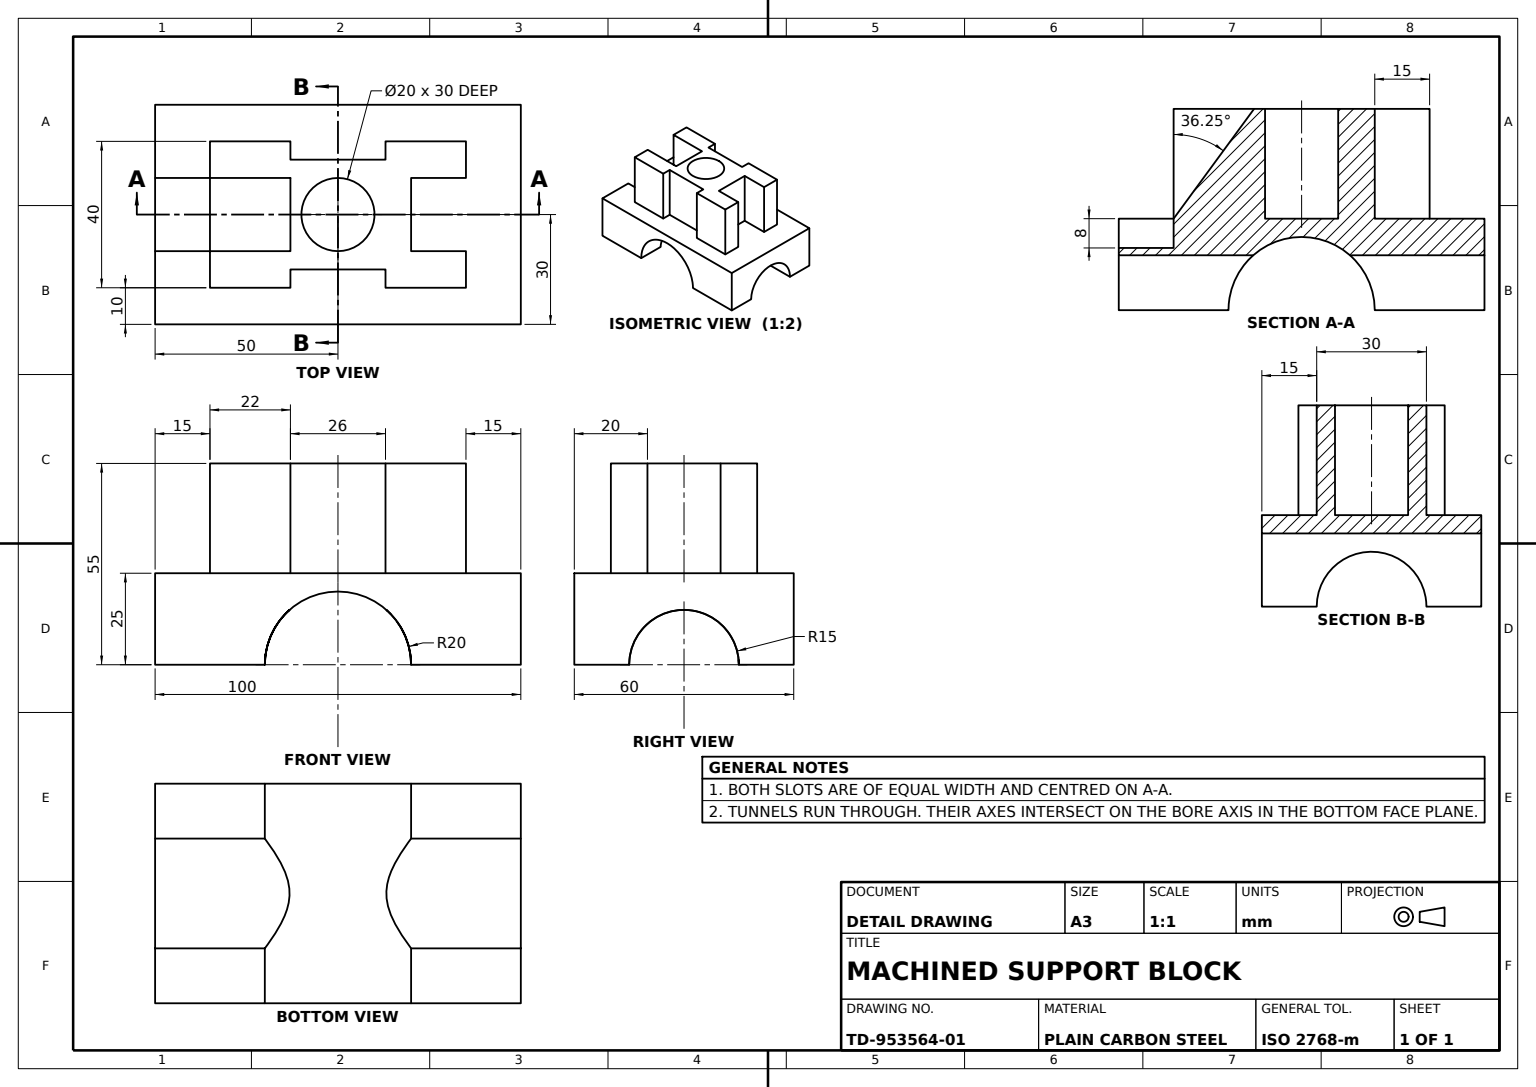
ISO-10303-21;
HEADER;
FILE_DESCRIPTION((''),'2;1');
FILE_NAME('','',(''),(''),'','','');
FILE_SCHEMA(('AUTOMOTIVE_DESIGN'));
ENDSEC;
DATA;
#1=APPLICATION_CONTEXT('');
#2=PRODUCT_CONTEXT('',#1,'mechanical');
#3=PRODUCT('','','',(#2));
#4=PRODUCT_DEFINITION_FORMATION('','',#3);
#5=PRODUCT_DEFINITION_CONTEXT('',#1,'design');
#6=PRODUCT_DEFINITION('','',#4,#5);
#7=PRODUCT_DEFINITION_SHAPE('','',#6);
#8=(LENGTH_UNIT()NAMED_UNIT(*)SI_UNIT(.MILLI.,.METRE.));
#9=(NAMED_UNIT(*)PLANE_ANGLE_UNIT()SI_UNIT($,.RADIAN.));
#10=(NAMED_UNIT(*)SI_UNIT($,.STERADIAN.)SOLID_ANGLE_UNIT());
#11=UNCERTAINTY_MEASURE_WITH_UNIT(LENGTH_MEASURE(1.E-05),#8,'distance_accuracy_value','');
#12=(GEOMETRIC_REPRESENTATION_CONTEXT(3)GLOBAL_UNCERTAINTY_ASSIGNED_CONTEXT((#11))GLOBAL_UNIT_ASSIGNED_CONTEXT((#8,#9,#10))REPRESENTATION_CONTEXT('',''));
#13=CARTESIAN_POINT('',(35.,42.5,20.));
#14=VERTEX_POINT('',#13);
#15=CARTESIAN_POINT('',(35.,12.5,20.));
#16=VERTEX_POINT('',#15);
#17=DIRECTION('',(0.,-1.,0.));
#18=VECTOR('',#17,1000.);
#19=LINE('',#13,#18);
#20=EDGE_CURVE('',#14,#16,#19,.T.);
#21=ORIENTED_EDGE('',*,*,#20,.F.);
#22=CARTESIAN_POINT('',(13.,42.5,20.));
#23=VERTEX_POINT('',#22);
#24=DIRECTION('',(1.,0.,0.));
#25=VECTOR('',#24,1000.);
#26=LINE('',#13,#25);
#27=EDGE_CURVE('',#23,#14,#26,.T.);
#28=ORIENTED_EDGE('',*,*,#27,.F.);
#29=CARTESIAN_POINT('',(13.,12.5,20.));
#30=VERTEX_POINT('',#29);
#31=LINE('',#22,#18);
#32=EDGE_CURVE('',#23,#30,#31,.T.);
#33=ORIENTED_EDGE('',*,*,#32,.T.);
#34=LINE('',#15,#25);
#35=EDGE_CURVE('',#30,#16,#34,.T.);
#36=ORIENTED_EDGE('',*,*,#35,.T.);
#37=EDGE_LOOP('',(#21,#28,#33,#36));
#38=FACE_OUTER_BOUND('',#37,.T.);
#39=DIRECTION('',(0.,0.,-1.));
#40=DIRECTION('',(-1.,0.,0.));
#41=AXIS2_PLACEMENT_3D('',#13,#39,#40);
#42=PLANE('',#41);
#43=ADVANCED_FACE('',(#38),#42,.F.);
#44=CARTESIAN_POINT('',(-35.,12.5,20.));
#45=VERTEX_POINT('',#44);
#46=CARTESIAN_POINT('',(-13.,12.5,20.));
#47=VERTEX_POINT('',#46);
#48=LINE('',#46,#25);
#49=EDGE_CURVE('',#45,#47,#48,.T.);
#50=ORIENTED_EDGE('',*,*,#49,.T.);
#51=CARTESIAN_POINT('',(-13.,42.5,20.));
#52=VERTEX_POINT('',#51);
#53=LINE('',#51,#18);
#54=EDGE_CURVE('',#52,#47,#53,.T.);
#55=ORIENTED_EDGE('',*,*,#54,.F.);
#56=CARTESIAN_POINT('',(-35.,42.5,20.));
#57=VERTEX_POINT('',#56);
#58=VECTOR('',#40,1000.);
#59=LINE('',#56,#58);
#60=EDGE_CURVE('',#52,#57,#59,.T.);
#61=ORIENTED_EDGE('',*,*,#60,.T.);
#62=LINE('',#44,#18);
#63=EDGE_CURVE('',#57,#45,#62,.T.);
#64=ORIENTED_EDGE('',*,*,#63,.T.);
#65=EDGE_LOOP('',(#50,#55,#61,#64));
#66=FACE_OUTER_BOUND('',#65,.T.);
#67=AXIS2_PLACEMENT_3D('',#51,#39,#40);
#68=PLANE('',#67);
#69=ADVANCED_FACE('',(#66),#68,.F.);
#70=CARTESIAN_POINT('',(35.,42.5,-10.));
#71=VERTEX_POINT('',#70);
#72=CARTESIAN_POINT('',(35.,12.5,-10.));
#73=VERTEX_POINT('',#72);
#74=LINE('',#70,#18);
#75=EDGE_CURVE('',#71,#73,#74,.T.);
#76=ORIENTED_EDGE('',*,*,#75,.F.);
#77=CARTESIAN_POINT('',(20.,42.5,-10.));
#78=VERTEX_POINT('',#77);
#79=LINE('',#77,#25);
#80=EDGE_CURVE('',#78,#71,#79,.T.);
#81=ORIENTED_EDGE('',*,*,#80,.F.);
#82=CARTESIAN_POINT('',(20.,12.5,-10.));
#83=VERTEX_POINT('',#82);
#84=LINE('',#77,#18);
#85=EDGE_CURVE('',#78,#83,#84,.T.);
#86=ORIENTED_EDGE('',*,*,#85,.T.);
#87=LINE('',#82,#25);
#88=EDGE_CURVE('',#83,#73,#87,.T.);
#89=ORIENTED_EDGE('',*,*,#88,.T.);
#90=EDGE_LOOP('',(#76,#81,#86,#89));
#91=FACE_OUTER_BOUND('',#90,.T.);
#92=AXIS2_PLACEMENT_3D('',#77,#39,#40);
#93=PLANE('',#92);
#94=ADVANCED_FACE('',(#91),#93,.F.);
#95=CARTESIAN_POINT('',(-20.,-12.5,30.));
#96=VERTEX_POINT('',#95);
#97=CARTESIAN_POINT('',(20.,-12.5,30.));
#98=VERTEX_POINT('',#97);
#99=CARTESIAN_POINT('',(0.,-12.5,30.));
#100=AXIS2_PLACEMENT_3D('',#99,#39,#24);
#101=CIRCLE('',#100,20.);
#102=EDGE_CURVE('',#96,#98,#101,.T.);
#103=ORIENTED_EDGE('',*,*,#102,.F.);
#104=CARTESIAN_POINT('',(-20.,-12.5,15.));
#105=VERTEX_POINT('',#104);
#106=VECTOR('',#39,1000.);
#107=LINE('',#95,#106);
#108=EDGE_CURVE('',#96,#105,#107,.T.);
#109=ORIENTED_EDGE('',*,*,#108,.T.);
#110=CARTESIAN_POINT('',(-20.,-12.5,-15.));
#111=VERTEX_POINT('',#110);
#112=CARTESIAN_POINT('',(-20.,-11.460012,15.));
#113=CARTESIAN_POINT('',(-19.91945,-10.444489,14.89307));
#114=CARTESIAN_POINT('',(-19.68971,-8.954901,14.583876));
#115=CARTESIAN_POINT('',(-19.594347,-8.461833,14.455074));
#116=CARTESIAN_POINT('',(-19.370481,-7.49703,14.150132));
#117=CARTESIAN_POINT('',(-19.243229,-7.02976,13.975697));
#118=CARTESIAN_POINT('',(-18.961995,-6.122842,13.585856));
#119=CARTESIAN_POINT('',(-18.807998,-5.683203,13.37044));
#120=CARTESIAN_POINT('',(-18.476456,-4.829922,12.899895));
#121=CARTESIAN_POINT('',(-18.297983,-4.414425,12.64341));
#122=CARTESIAN_POINT('',(-17.739419,-3.221867,11.825632));
#123=CARTESIAN_POINT('',(-17.337061,-2.498089,11.218166));
#124=CARTESIAN_POINT('',(-16.711435,-1.505414,10.214717));
#125=CARTESIAN_POINT('',(-16.498395,-1.18907,9.863302));
#126=CARTESIAN_POINT('',(-16.073156,-0.592531,9.134223));
#127=CARTESIAN_POINT('',(-15.861739,-0.31326,8.758001));
#128=CARTESIAN_POINT('',(-15.238528,0.470461,7.592364));
#129=CARTESIAN_POINT('',(-14.836864,0.921647,6.766908));
#130=CARTESIAN_POINT('',(-14.29593,1.489091,5.434909));
#131=CARTESIAN_POINT('',(-14.125386,1.660451,4.972426));
#132=CARTESIAN_POINT('',(-13.822168,1.956576,4.031229));
#133=CARTESIAN_POINT('',(-13.688686,2.082271,3.550951));
#134=CARTESIAN_POINT('',(-13.467259,2.28701,2.568307));
#135=CARTESIAN_POINT('',(-13.379218,2.366168,2.065023));
#136=CARTESIAN_POINT('',(-13.259474,2.473069,1.036579));
#137=CARTESIAN_POINT('',(-13.22921,2.4996,0.523513));
#138=CARTESIAN_POINT('',(-13.228313,2.500391,-0.500332));
#139=CARTESIAN_POINT('',(-13.257676,2.474649,-1.011111));
#140=CARTESIAN_POINT('',(-13.374088,2.370772,-2.030418));
#141=CARTESIAN_POINT('',(-13.461925,2.291862,-2.540716));
#142=CARTESIAN_POINT('',(-13.682828,2.087763,-3.528684));
#143=CARTESIAN_POINT('',(-13.816081,1.962383,-4.010379));
#144=CARTESIAN_POINT('',(-14.118367,1.667438,-4.952509));
#145=CARTESIAN_POINT('',(-14.288407,1.496778,-5.415214));
#146=CARTESIAN_POINT('',(-14.829898,0.929354,-6.752021));
#147=CARTESIAN_POINT('',(-15.232138,0.477984,-7.579673));
#148=CARTESIAN_POINT('',(-15.856074,-0.305885,-8.747768));
#149=CARTESIAN_POINT('',(-16.067715,-0.585187,-9.124663));
#150=CARTESIAN_POINT('',(-16.493336,-1.181692,-9.854854));
#151=CARTESIAN_POINT('',(-16.706461,-1.497879,-10.206576));
#152=CARTESIAN_POINT('',(-17.331547,-2.488635,-11.209639));
#153=CARTESIAN_POINT('',(-17.73267,-3.209534,-11.815456));
#154=CARTESIAN_POINT('',(-18.288634,-4.393461,-12.629864));
#155=CARTESIAN_POINT('',(-18.466869,-4.806673,-12.886183));
#156=CARTESIAN_POINT('',(-18.801726,-5.665702,-13.361638));
#157=CARTESIAN_POINT('',(-18.956617,-6.106875,-13.578352));
#158=CARTESIAN_POINT('',(-19.238591,-7.013474,-13.969314));
#159=CARTESIAN_POINT('',(-19.365686,-7.478895,-14.143566));
#160=CARTESIAN_POINT('',(-19.588837,-8.435671,-14.447602));
#161=CARTESIAN_POINT('',(-19.685272,-8.929505,-14.57789));
#162=CARTESIAN_POINT('',(-19.91921,-10.436366,-14.892772));
#163=CARTESIAN_POINT('',(-20.,-11.458775,-15.));
#164=B_SPLINE_CURVE_WITH_KNOTS('',3,(#104,#112,#113,#114,#115,#116,#117,#118,#119,#120,#121,#122,#123,#124,#125,#126,#127,#128,#129,#130,#131,#132,#133,#134,#135,#136,#137,#138,#139,#140,#141,#142,#143,#144,#145,#146,#147,#148,#149,#150,#151,#152,#153,#154,#155,#156,#157,#158,#159,#160,#161,#162,#163,#110),.UNSPECIFIED.,.F.,.F.,(4,2,2,2,2,2,2,2,2,2,2,2,2,2,2,2,2,2,2,2,2,2,2,2,2,2,4),(0.,0.003069136,0.004603704,0.006138272,0.00767284,0.009207408,0.012276544,0.013811112,0.01534568,0.018414816,0.019949384,0.021483952,0.02301852,0.024553088,0.026087656,0.027622224,0.029156792,0.03069136,0.033760496,0.035295064,0.036829632,0.039898768,0.041433336,0.042967904,0.044502472,0.04603704,0.049106176),.UNSPECIFIED.);
#165=EDGE_CURVE('',#105,#111,#164,.T.);
#166=ORIENTED_EDGE('',*,*,#165,.T.);
#167=CARTESIAN_POINT('',(-20.,-12.5,-30.));
#168=VERTEX_POINT('',#167);
#169=EDGE_CURVE('',#111,#168,#107,.T.);
#170=ORIENTED_EDGE('',*,*,#169,.T.);
#171=CARTESIAN_POINT('',(20.,-12.5,-30.));
#172=VERTEX_POINT('',#171);
#173=CARTESIAN_POINT('',(0.,-12.5,-30.));
#174=AXIS2_PLACEMENT_3D('',#173,#39,#24);
#175=CIRCLE('',#174,20.);
#176=EDGE_CURVE('',#168,#172,#175,.T.);
#177=ORIENTED_EDGE('',*,*,#176,.T.);
#178=CARTESIAN_POINT('',(20.,-12.5,-15.));
#179=VERTEX_POINT('',#178);
#180=LINE('',#97,#106);
#181=EDGE_CURVE('',#179,#172,#180,.T.);
#182=ORIENTED_EDGE('',*,*,#181,.F.);
#183=CARTESIAN_POINT('',(20.,-12.5,15.));
#184=VERTEX_POINT('',#183);
#185=CARTESIAN_POINT('',(20.,-11.460012,-15.));
#186=CARTESIAN_POINT('',(19.91945,-10.444489,-14.89307));
#187=CARTESIAN_POINT('',(19.68971,-8.954901,-14.583876));
#188=CARTESIAN_POINT('',(19.594347,-8.461833,-14.455074));
#189=CARTESIAN_POINT('',(19.370481,-7.49703,-14.150132));
#190=CARTESIAN_POINT('',(19.243229,-7.02976,-13.975697));
#191=CARTESIAN_POINT('',(18.961995,-6.122842,-13.585856));
#192=CARTESIAN_POINT('',(18.807998,-5.683203,-13.37044));
#193=CARTESIAN_POINT('',(18.476456,-4.829922,-12.899895));
#194=CARTESIAN_POINT('',(18.297983,-4.414425,-12.64341));
#195=CARTESIAN_POINT('',(17.739419,-3.221867,-11.825632));
#196=CARTESIAN_POINT('',(17.337061,-2.498089,-11.218166));
#197=CARTESIAN_POINT('',(16.711435,-1.505414,-10.214717));
#198=CARTESIAN_POINT('',(16.498395,-1.18907,-9.863302));
#199=CARTESIAN_POINT('',(16.073156,-0.592531,-9.134223));
#200=CARTESIAN_POINT('',(15.861739,-0.31326,-8.758001));
#201=CARTESIAN_POINT('',(15.238528,0.470461,-7.592364));
#202=CARTESIAN_POINT('',(14.836864,0.921647,-6.766908));
#203=CARTESIAN_POINT('',(14.29593,1.489091,-5.434909));
#204=CARTESIAN_POINT('',(14.125386,1.660451,-4.972426));
#205=CARTESIAN_POINT('',(13.822168,1.956576,-4.031229));
#206=CARTESIAN_POINT('',(13.688686,2.082271,-3.550951));
#207=CARTESIAN_POINT('',(13.467259,2.28701,-2.568307));
#208=CARTESIAN_POINT('',(13.379218,2.366168,-2.065023));
#209=CARTESIAN_POINT('',(13.259474,2.473069,-1.036579));
#210=CARTESIAN_POINT('',(13.22921,2.4996,-0.523513));
#211=CARTESIAN_POINT('',(13.228313,2.500391,0.500332));
#212=CARTESIAN_POINT('',(13.257676,2.474649,1.011111));
#213=CARTESIAN_POINT('',(13.374088,2.370772,2.030418));
#214=CARTESIAN_POINT('',(13.461925,2.291862,2.540716));
#215=CARTESIAN_POINT('',(13.682828,2.087763,3.528684));
#216=CARTESIAN_POINT('',(13.816081,1.962383,4.010379));
#217=CARTESIAN_POINT('',(14.118367,1.667438,4.952509));
#218=CARTESIAN_POINT('',(14.288407,1.496778,5.415214));
#219=CARTESIAN_POINT('',(14.829898,0.929354,6.752021));
#220=CARTESIAN_POINT('',(15.232138,0.477984,7.579673));
#221=CARTESIAN_POINT('',(15.856074,-0.305885,8.747768));
#222=CARTESIAN_POINT('',(16.067715,-0.585187,9.124663));
#223=CARTESIAN_POINT('',(16.493336,-1.181692,9.854854));
#224=CARTESIAN_POINT('',(16.706461,-1.497879,10.206576));
#225=CARTESIAN_POINT('',(17.331547,-2.488635,11.209639));
#226=CARTESIAN_POINT('',(17.73267,-3.209534,11.815456));
#227=CARTESIAN_POINT('',(18.288634,-4.393461,12.629864));
#228=CARTESIAN_POINT('',(18.466869,-4.806673,12.886183));
#229=CARTESIAN_POINT('',(18.801726,-5.665702,13.361638));
#230=CARTESIAN_POINT('',(18.956617,-6.106875,13.578352));
#231=CARTESIAN_POINT('',(19.238591,-7.013474,13.969314));
#232=CARTESIAN_POINT('',(19.365686,-7.478895,14.143566));
#233=CARTESIAN_POINT('',(19.588837,-8.435671,14.447602));
#234=CARTESIAN_POINT('',(19.685272,-8.929505,14.57789));
#235=CARTESIAN_POINT('',(19.91921,-10.436366,14.892772));
#236=CARTESIAN_POINT('',(20.,-11.458775,15.));
#237=B_SPLINE_CURVE_WITH_KNOTS('',3,(#178,#185,#186,#187,#188,#189,#190,#191,#192,#193,#194,#195,#196,#197,#198,#199,#200,#201,#202,#203,#204,#205,#206,#207,#208,#209,#210,#211,#212,#213,#214,#215,#216,#217,#218,#219,#220,#221,#222,#223,#224,#225,#226,#227,#228,#229,#230,#231,#232,#233,#234,#235,#236,#183),.UNSPECIFIED.,.F.,.F.,(4,2,2,2,2,2,2,2,2,2,2,2,2,2,2,2,2,2,2,2,2,2,2,2,2,2,4),(0.,0.003069136,0.004603704,0.006138272,0.00767284,0.009207408,0.012276544,0.013811112,0.01534568,0.018414816,0.019949384,0.021483952,0.02301852,0.024553088,0.026087656,0.027622224,0.029156792,0.03069136,0.033760496,0.035295064,0.036829632,0.039898768,0.041433336,0.042967904,0.044502472,0.04603704,0.049106176),.UNSPECIFIED.);
#238=EDGE_CURVE('',#179,#184,#237,.T.);
#239=ORIENTED_EDGE('',*,*,#238,.T.);
#240=EDGE_CURVE('',#98,#184,#180,.T.);
#241=ORIENTED_EDGE('',*,*,#240,.F.);
#242=EDGE_LOOP('',(#103,#109,#166,#170,#177,#182,#239,#241));
#243=FACE_OUTER_BOUND('',#242,.T.);
#244=AXIS2_PLACEMENT_3D('',#99,#39,#40);
#245=CYLINDRICAL_SURFACE('',#244,20.);
#246=ADVANCED_FACE('',(#243),#245,.F.);
#247=CARTESIAN_POINT('',(-13.,42.5,-20.));
#248=VERTEX_POINT('',#247);
#249=CARTESIAN_POINT('',(-13.,12.5,-20.));
#250=VERTEX_POINT('',#249);
#251=LINE('',#247,#18);
#252=EDGE_CURVE('',#248,#250,#251,.T.);
#253=ORIENTED_EDGE('',*,*,#252,.T.);
#254=CARTESIAN_POINT('',(-35.,12.5,-20.));
#255=VERTEX_POINT('',#254);
#256=LINE('',#249,#58);
#257=EDGE_CURVE('',#250,#255,#256,.T.);
#258=ORIENTED_EDGE('',*,*,#257,.T.);
#259=CARTESIAN_POINT('',(-35.,42.5,-20.));
#260=VERTEX_POINT('',#259);
#261=LINE('',#259,#18);
#262=EDGE_CURVE('',#260,#255,#261,.T.);
#263=ORIENTED_EDGE('',*,*,#262,.F.);
#264=LINE('',#247,#58);
#265=EDGE_CURVE('',#248,#260,#264,.T.);
#266=ORIENTED_EDGE('',*,*,#265,.F.);
#267=EDGE_LOOP('',(#253,#258,#263,#266));
#268=FACE_OUTER_BOUND('',#267,.T.);
#269=DIRECTION('',(0.,0.,1.));
#270=AXIS2_PLACEMENT_3D('',#247,#269,#24);
#271=PLANE('',#270);
#272=ADVANCED_FACE('',(#268),#271,.F.);
#273=CARTESIAN_POINT('',(-13.,42.5,15.));
#274=VERTEX_POINT('',#273);
#275=CARTESIAN_POINT('',(13.,42.5,15.));
#276=VERTEX_POINT('',#275);
#277=LINE('',#275,#25);
#278=EDGE_CURVE('',#274,#276,#277,.T.);
#279=ORIENTED_EDGE('',*,*,#278,.F.);
#280=CARTESIAN_POINT('',(-13.,12.5,15.));
#281=VERTEX_POINT('',#280);
#282=LINE('',#273,#18);
#283=EDGE_CURVE('',#274,#281,#282,.T.);
#284=ORIENTED_EDGE('',*,*,#283,.T.);
#285=CARTESIAN_POINT('',(13.,12.5,15.));
#286=VERTEX_POINT('',#285);
#287=LINE('',#285,#25);
#288=EDGE_CURVE('',#281,#286,#287,.T.);
#289=ORIENTED_EDGE('',*,*,#288,.T.);
#290=LINE('',#275,#18);
#291=EDGE_CURVE('',#276,#286,#290,.T.);
#292=ORIENTED_EDGE('',*,*,#291,.F.);
#293=EDGE_LOOP('',(#279,#284,#289,#292));
#294=FACE_OUTER_BOUND('',#293,.T.);
#295=AXIS2_PLACEMENT_3D('',#275,#39,#40);
#296=PLANE('',#295);
#297=ADVANCED_FACE('',(#294),#296,.F.);
#298=CARTESIAN_POINT('',(50.,-12.5,30.));
#299=VERTEX_POINT('',#298);
#300=CARTESIAN_POINT('',(50.,12.5,30.));
#301=VERTEX_POINT('',#300);
#302=DIRECTION('',(0.,1.,0.));
#303=VECTOR('',#302,1000.);
#304=LINE('',#300,#303);
#305=EDGE_CURVE('',#299,#301,#304,.T.);
#306=ORIENTED_EDGE('',*,*,#305,.T.);
#307=CARTESIAN_POINT('',(-50.,12.5,30.));
#308=VERTEX_POINT('',#307);
#309=LINE('',#307,#58);
#310=EDGE_CURVE('',#301,#308,#309,.T.);
#311=ORIENTED_EDGE('',*,*,#310,.T.);
#312=CARTESIAN_POINT('',(-50.,-12.5,30.));
#313=VERTEX_POINT('',#312);
#314=LINE('',#307,#18);
#315=EDGE_CURVE('',#308,#313,#314,.T.);
#316=ORIENTED_EDGE('',*,*,#315,.T.);
#317=LINE('',#312,#25);
#318=EDGE_CURVE('',#313,#96,#317,.T.);
#319=ORIENTED_EDGE('',*,*,#318,.T.);
#320=ORIENTED_EDGE('',*,*,#102,.T.);
#321=LINE('',#97,#25);
#322=EDGE_CURVE('',#98,#299,#321,.T.);
#323=ORIENTED_EDGE('',*,*,#322,.T.);
#324=EDGE_LOOP('',(#306,#311,#316,#319,#320,#323));
#325=FACE_OUTER_BOUND('',#324,.T.);
#326=AXIS2_PLACEMENT_3D('',#99,#269,#24);
#327=PLANE('',#326);
#328=ADVANCED_FACE('',(#325),#327,.T.);
#329=CARTESIAN_POINT('',(35.,12.5,-20.));
#330=VERTEX_POINT('',#329);
#331=LINE('',#72,#106);
#332=EDGE_CURVE('',#73,#330,#331,.T.);
#333=ORIENTED_EDGE('',*,*,#332,.T.);
#334=CARTESIAN_POINT('',(35.,42.5,-20.));
#335=VERTEX_POINT('',#334);
#336=LINE('',#334,#18);
#337=EDGE_CURVE('',#335,#330,#336,.T.);
#338=ORIENTED_EDGE('',*,*,#337,.F.);
#339=LINE('',#70,#106);
#340=EDGE_CURVE('',#71,#335,#339,.T.);
#341=ORIENTED_EDGE('',*,*,#340,.F.);
#342=ORIENTED_EDGE('',*,*,#75,.T.);
#343=EDGE_LOOP('',(#333,#338,#341,#342));
#344=FACE_OUTER_BOUND('',#343,.T.);
#345=AXIS2_PLACEMENT_3D('',#70,#40,#269);
#346=PLANE('',#345);
#347=ADVANCED_FACE('',(#344),#346,.F.);
#348=ORIENTED_EDGE('',*,*,#165,.F.);
#349=CARTESIAN_POINT('',(-50.,-12.5,15.));
#350=VERTEX_POINT('',#349);
#351=CARTESIAN_POINT('',(50.,-12.5,15.));
#352=LINE('',#351,#58);
#353=EDGE_CURVE('',#105,#350,#352,.T.);
#354=ORIENTED_EDGE('',*,*,#353,.T.);
#355=CARTESIAN_POINT('',(-50.,-12.5,-15.));
#356=VERTEX_POINT('',#355);
#357=CARTESIAN_POINT('',(-50.,-12.5,0.));
#358=AXIS2_PLACEMENT_3D('',#357,#40,#269);
#359=CIRCLE('',#358,15.);
#360=EDGE_CURVE('',#350,#356,#359,.T.);
#361=ORIENTED_EDGE('',*,*,#360,.T.);
#362=CARTESIAN_POINT('',(50.,-12.5,-15.));
#363=LINE('',#362,#58);
#364=EDGE_CURVE('',#111,#356,#363,.T.);
#365=ORIENTED_EDGE('',*,*,#364,.F.);
#366=EDGE_LOOP('',(#348,#354,#361,#365));
#367=FACE_OUTER_BOUND('',#366,.T.);
#368=CARTESIAN_POINT('',(50.,-12.5,0.));
#369=AXIS2_PLACEMENT_3D('',#368,#40,#269);
#370=CYLINDRICAL_SURFACE('',#369,15.);
#371=ADVANCED_FACE('',(#367),#370,.F.);
#372=ORIENTED_EDGE('',*,*,#20,.T.);
#373=CARTESIAN_POINT('',(35.,12.5,10.));
#374=VERTEX_POINT('',#373);
#375=LINE('',#373,#106);
#376=EDGE_CURVE('',#16,#374,#375,.T.);
#377=ORIENTED_EDGE('',*,*,#376,.T.);
#378=CARTESIAN_POINT('',(35.,42.5,10.));
#379=VERTEX_POINT('',#378);
#380=LINE('',#378,#18);
#381=EDGE_CURVE('',#379,#374,#380,.T.);
#382=ORIENTED_EDGE('',*,*,#381,.F.);
#383=LINE('',#378,#106);
#384=EDGE_CURVE('',#14,#379,#383,.T.);
#385=ORIENTED_EDGE('',*,*,#384,.F.);
#386=EDGE_LOOP('',(#372,#377,#382,#385));
#387=FACE_OUTER_BOUND('',#386,.T.);
#388=AXIS2_PLACEMENT_3D('',#378,#40,#269);
#389=PLANE('',#388);
#390=ADVANCED_FACE('',(#387),#389,.F.);
#391=CARTESIAN_POINT('',(-35.,12.5,-10.));
#392=VERTEX_POINT('',#391);
#393=CARTESIAN_POINT('',(-35.,4.5,-10.));
#394=VERTEX_POINT('',#393);
#395=LINE('',#393,#18);
#396=EDGE_CURVE('',#392,#394,#395,.T.);
#397=ORIENTED_EDGE('',*,*,#396,.F.);
#398=CARTESIAN_POINT('',(-50.,12.5,-10.));
#399=VERTEX_POINT('',#398);
#400=LINE('',#391,#58);
#401=EDGE_CURVE('',#392,#399,#400,.T.);
#402=ORIENTED_EDGE('',*,*,#401,.T.);
#403=CARTESIAN_POINT('',(-50.,4.5,-10.));
#404=VERTEX_POINT('',#403);
#405=LINE('',#403,#18);
#406=EDGE_CURVE('',#399,#404,#405,.T.);
#407=ORIENTED_EDGE('',*,*,#406,.T.);
#408=LINE('',#393,#58);
#409=EDGE_CURVE('',#394,#404,#408,.T.);
#410=ORIENTED_EDGE('',*,*,#409,.F.);
#411=EDGE_LOOP('',(#397,#402,#407,#410));
#412=FACE_OUTER_BOUND('',#411,.T.);
#413=AXIS2_PLACEMENT_3D('',#393,#39,#302);
#414=PLANE('',#413);
#415=ADVANCED_FACE('',(#412),#414,.F.);
#416=CARTESIAN_POINT('',(0.,42.5,10.));
#417=VERTEX_POINT('',#416);
#418=CARTESIAN_POINT('',(0.,42.5,-10.));
#419=VERTEX_POINT('',#418);
#420=CARTESIAN_POINT('',(0.,42.5,0.));
#421=AXIS2_PLACEMENT_3D('',#420,#302,#269);
#422=CIRCLE('',#421,10.);
#423=EDGE_CURVE('',#417,#419,#422,.T.);
#424=ORIENTED_EDGE('',*,*,#423,.F.);
#425=EDGE_CURVE('',#419,#417,#422,.T.);
#426=ORIENTED_EDGE('',*,*,#425,.F.);
#427=EDGE_LOOP('',(#424,#426));
#428=FACE_BOUND('',#427,.T.);
#429=CARTESIAN_POINT('',(20.,42.5,10.));
#430=VERTEX_POINT('',#429);
#431=LINE('',#429,#58);
#432=EDGE_CURVE('',#379,#430,#431,.T.);
#433=ORIENTED_EDGE('',*,*,#432,.T.);
#434=LINE('',#429,#106);
#435=EDGE_CURVE('',#430,#78,#434,.T.);
#436=ORIENTED_EDGE('',*,*,#435,.T.);
#437=ORIENTED_EDGE('',*,*,#80,.T.);
#438=ORIENTED_EDGE('',*,*,#340,.T.);
#439=CARTESIAN_POINT('',(13.,42.5,-20.));
#440=VERTEX_POINT('',#439);
#441=LINE('',#334,#58);
#442=EDGE_CURVE('',#335,#440,#441,.T.);
#443=ORIENTED_EDGE('',*,*,#442,.T.);
#444=CARTESIAN_POINT('',(13.,42.5,-15.));
#445=VERTEX_POINT('',#444);
#446=VECTOR('',#269,1000.);
#447=LINE('',#439,#446);
#448=EDGE_CURVE('',#440,#445,#447,.T.);
#449=ORIENTED_EDGE('',*,*,#448,.T.);
#450=CARTESIAN_POINT('',(-13.,42.5,-15.));
#451=VERTEX_POINT('',#450);
#452=LINE('',#444,#58);
#453=EDGE_CURVE('',#445,#451,#452,.T.);
#454=ORIENTED_EDGE('',*,*,#453,.T.);
#455=LINE('',#450,#106);
#456=EDGE_CURVE('',#451,#248,#455,.T.);
#457=ORIENTED_EDGE('',*,*,#456,.T.);
#458=ORIENTED_EDGE('',*,*,#265,.T.);
#459=CARTESIAN_POINT('',(-35.,42.5,-10.));
#460=VERTEX_POINT('',#459);
#461=LINE('',#259,#446);
#462=EDGE_CURVE('',#260,#460,#461,.T.);
#463=ORIENTED_EDGE('',*,*,#462,.T.);
#464=CARTESIAN_POINT('',(-13.,42.5,-10.));
#465=VERTEX_POINT('',#464);
#466=LINE('',#464,#58);
#467=EDGE_CURVE('',#465,#460,#466,.T.);
#468=ORIENTED_EDGE('',*,*,#467,.F.);
#469=CARTESIAN_POINT('',(-13.,42.5,10.));
#470=VERTEX_POINT('',#469);
#471=LINE('',#464,#446);
#472=EDGE_CURVE('',#465,#470,#471,.T.);
#473=ORIENTED_EDGE('',*,*,#472,.T.);
#474=CARTESIAN_POINT('',(-35.,42.5,10.));
#475=VERTEX_POINT('',#474);
#476=LINE('',#474,#58);
#477=EDGE_CURVE('',#470,#475,#476,.T.);
#478=ORIENTED_EDGE('',*,*,#477,.T.);
#479=LINE('',#474,#446);
#480=EDGE_CURVE('',#475,#57,#479,.T.);
#481=ORIENTED_EDGE('',*,*,#480,.T.);
#482=ORIENTED_EDGE('',*,*,#60,.F.);
#483=LINE('',#273,#106);
#484=EDGE_CURVE('',#52,#274,#483,.T.);
#485=ORIENTED_EDGE('',*,*,#484,.T.);
#486=ORIENTED_EDGE('',*,*,#278,.T.);
#487=LINE('',#22,#446);
#488=EDGE_CURVE('',#276,#23,#487,.T.);
#489=ORIENTED_EDGE('',*,*,#488,.T.);
#490=ORIENTED_EDGE('',*,*,#27,.T.);
#491=ORIENTED_EDGE('',*,*,#384,.T.);
#492=EDGE_LOOP('',(#433,#436,#437,#438,#443,#449,#454,#457,#458,#463,#468,#473,#478,#481,#482,#485,#486,#489,#490,#491));
#493=FACE_OUTER_BOUND('',#492,.T.);
#494=PLANE('',#421);
#495=ADVANCED_FACE('',(#428,#493),#494,.T.);
#496=CARTESIAN_POINT('',(-35.,12.5,10.));
#497=VERTEX_POINT('',#496);
#498=LINE('',#391,#446);
#499=EDGE_CURVE('',#392,#497,#498,.T.);
#500=ORIENTED_EDGE('',*,*,#499,.T.);
#501=DIRECTION('',(0.591363664,0.806404996,0.));
#502=VECTOR('',#501,1000.);
#503=LINE('',#469,#502);
#504=EDGE_CURVE('',#497,#470,#503,.T.);
#505=ORIENTED_EDGE('',*,*,#504,.T.);
#506=ORIENTED_EDGE('',*,*,#472,.F.);
#507=LINE('',#391,#502);
#508=EDGE_CURVE('',#392,#465,#507,.T.);
#509=ORIENTED_EDGE('',*,*,#508,.F.);
#510=EDGE_LOOP('',(#500,#505,#506,#509));
#511=FACE_OUTER_BOUND('',#510,.T.);
#512=DIRECTION('',(0.806404996,-0.591363664,0.));
#513=AXIS2_PLACEMENT_3D('',#391,#512,#501);
#514=PLANE('',#513);
#515=ADVANCED_FACE('',(#511),#514,.F.);
#516=ORIENTED_EDGE('',*,*,#364,.T.);
#517=CARTESIAN_POINT('',(-50.,-12.5,-30.));
#518=VERTEX_POINT('',#517);
#519=LINE('',#312,#106);
#520=EDGE_CURVE('',#356,#518,#519,.T.);
#521=ORIENTED_EDGE('',*,*,#520,.T.);
#522=LINE('',#517,#25);
#523=EDGE_CURVE('',#518,#168,#522,.T.);
#524=ORIENTED_EDGE('',*,*,#523,.T.);
#525=ORIENTED_EDGE('',*,*,#169,.F.);
#526=EDGE_LOOP('',(#516,#521,#524,#525));
#527=FACE_OUTER_BOUND('',#526,.T.);
#528=AXIS2_PLACEMENT_3D('',#312,#302,#269);
#529=PLANE('',#528);
#530=ADVANCED_FACE('',(#527),#529,.F.);
#531=ORIENTED_EDGE('',*,*,#360,.F.);
#532=EDGE_CURVE('',#313,#350,#519,.T.);
#533=ORIENTED_EDGE('',*,*,#532,.F.);
#534=ORIENTED_EDGE('',*,*,#315,.F.);
#535=CARTESIAN_POINT('',(-50.,12.5,10.));
#536=VERTEX_POINT('',#535);
#537=LINE('',#307,#106);
#538=EDGE_CURVE('',#308,#536,#537,.T.);
#539=ORIENTED_EDGE('',*,*,#538,.T.);
#540=CARTESIAN_POINT('',(-50.,4.5,10.));
#541=VERTEX_POINT('',#540);
#542=LINE('',#535,#303);
#543=EDGE_CURVE('',#541,#536,#542,.T.);
#544=ORIENTED_EDGE('',*,*,#543,.F.);
#545=LINE('',#540,#446);
#546=EDGE_CURVE('',#404,#541,#545,.T.);
#547=ORIENTED_EDGE('',*,*,#546,.F.);
#548=ORIENTED_EDGE('',*,*,#406,.F.);
#549=CARTESIAN_POINT('',(-50.,12.5,-30.));
#550=VERTEX_POINT('',#549);
#551=EDGE_CURVE('',#399,#550,#537,.T.);
#552=ORIENTED_EDGE('',*,*,#551,.T.);
#553=LINE('',#549,#18);
#554=EDGE_CURVE('',#550,#518,#553,.T.);
#555=ORIENTED_EDGE('',*,*,#554,.T.);
#556=ORIENTED_EDGE('',*,*,#520,.F.);
#557=EDGE_LOOP('',(#531,#533,#534,#539,#544,#547,#548,#552,#555,#556));
#558=FACE_OUTER_BOUND('',#557,.T.);
#559=AXIS2_PLACEMENT_3D('',#307,#24,#39);
#560=PLANE('',#559);
#561=ADVANCED_FACE('',(#558),#560,.F.);
#562=ORIENTED_EDGE('',*,*,#337,.T.);
#563=CARTESIAN_POINT('',(13.,12.5,-20.));
#564=VERTEX_POINT('',#563);
#565=LINE('',#329,#58);
#566=EDGE_CURVE('',#330,#564,#565,.T.);
#567=ORIENTED_EDGE('',*,*,#566,.T.);
#568=LINE('',#439,#18);
#569=EDGE_CURVE('',#440,#564,#568,.T.);
#570=ORIENTED_EDGE('',*,*,#569,.F.);
#571=ORIENTED_EDGE('',*,*,#442,.F.);
#572=EDGE_LOOP('',(#562,#567,#570,#571));
#573=FACE_OUTER_BOUND('',#572,.T.);
#574=AXIS2_PLACEMENT_3D('',#334,#269,#24);
#575=PLANE('',#574);
#576=ADVANCED_FACE('',(#573),#575,.F.);
#577=VERTEX_POINT('',#362);
#578=CARTESIAN_POINT('',(50.,-12.5,-30.));
#579=VERTEX_POINT('',#578);
#580=LINE('',#298,#106);
#581=EDGE_CURVE('',#577,#579,#580,.T.);
#582=ORIENTED_EDGE('',*,*,#581,.F.);
#583=EDGE_CURVE('',#577,#179,#363,.T.);
#584=ORIENTED_EDGE('',*,*,#583,.T.);
#585=ORIENTED_EDGE('',*,*,#181,.T.);
#586=LINE('',#171,#25);
#587=EDGE_CURVE('',#172,#579,#586,.T.);
#588=ORIENTED_EDGE('',*,*,#587,.T.);
#589=EDGE_LOOP('',(#582,#584,#585,#588));
#590=FACE_OUTER_BOUND('',#589,.T.);
#591=AXIS2_PLACEMENT_3D('',#97,#302,#269);
#592=PLANE('',#591);
#593=ADVANCED_FACE('',(#590),#592,.F.);
#594=CARTESIAN_POINT('',(-35.,4.5,10.));
#595=VERTEX_POINT('',#594);
#596=LINE('',#594,#58);
#597=EDGE_CURVE('',#595,#541,#596,.T.);
#598=ORIENTED_EDGE('',*,*,#597,.F.);
#599=LINE('',#594,#446);
#600=EDGE_CURVE('',#394,#595,#599,.T.);
#601=ORIENTED_EDGE('',*,*,#600,.F.);
#602=ORIENTED_EDGE('',*,*,#409,.T.);
#603=ORIENTED_EDGE('',*,*,#546,.T.);
#604=EDGE_LOOP('',(#598,#601,#602,#603));
#605=FACE_OUTER_BOUND('',#604,.T.);
#606=AXIS2_PLACEMENT_3D('',#594,#17,#39);
#607=PLANE('',#606);
#608=ADVANCED_FACE('',(#605),#607,.F.);
#609=ORIENTED_EDGE('',*,*,#252,.F.);
#610=ORIENTED_EDGE('',*,*,#456,.F.);
#611=CARTESIAN_POINT('',(-13.,12.5,-15.));
#612=VERTEX_POINT('',#611);
#613=LINE('',#450,#18);
#614=EDGE_CURVE('',#451,#612,#613,.T.);
#615=ORIENTED_EDGE('',*,*,#614,.T.);
#616=LINE('',#611,#106);
#617=EDGE_CURVE('',#612,#250,#616,.T.);
#618=ORIENTED_EDGE('',*,*,#617,.T.);
#619=EDGE_LOOP('',(#609,#610,#615,#618));
#620=FACE_OUTER_BOUND('',#619,.T.);
#621=AXIS2_PLACEMENT_3D('',#450,#40,#269);
#622=PLANE('',#621);
#623=ADVANCED_FACE('',(#620),#622,.F.);
#624=ORIENTED_EDGE('',*,*,#583,.F.);
#625=VERTEX_POINT('',#351);
#626=CIRCLE('',#369,15.);
#627=EDGE_CURVE('',#625,#577,#626,.T.);
#628=ORIENTED_EDGE('',*,*,#627,.F.);
#629=EDGE_CURVE('',#625,#184,#352,.T.);
#630=ORIENTED_EDGE('',*,*,#629,.T.);
#631=ORIENTED_EDGE('',*,*,#238,.F.);
#632=EDGE_LOOP('',(#624,#628,#630,#631));
#633=FACE_OUTER_BOUND('',#632,.T.);
#634=ADVANCED_FACE('',(#633),#370,.F.);
#635=CARTESIAN_POINT('',(20.,12.5,10.));
#636=VERTEX_POINT('',#635);
#637=LINE('',#635,#106);
#638=EDGE_CURVE('',#636,#83,#637,.T.);
#639=ORIENTED_EDGE('',*,*,#638,.T.);
#640=ORIENTED_EDGE('',*,*,#85,.F.);
#641=ORIENTED_EDGE('',*,*,#435,.F.);
#642=LINE('',#429,#18);
#643=EDGE_CURVE('',#430,#636,#642,.T.);
#644=ORIENTED_EDGE('',*,*,#643,.T.);
#645=EDGE_LOOP('',(#639,#640,#641,#644));
#646=FACE_OUTER_BOUND('',#645,.T.);
#647=AXIS2_PLACEMENT_3D('',#429,#40,#269);
#648=PLANE('',#647);
#649=ADVANCED_FACE('',(#646),#648,.F.);
#650=CARTESIAN_POINT('',(0.,12.5,10.));
#651=VERTEX_POINT('',#650);
#652=CARTESIAN_POINT('',(0.,12.5,-10.));
#653=VERTEX_POINT('',#652);
#654=CARTESIAN_POINT('',(0.,12.5,0.));
#655=AXIS2_PLACEMENT_3D('',#654,#302,#269);
#656=CIRCLE('',#655,10.);
#657=EDGE_CURVE('',#651,#653,#656,.T.);
#658=ORIENTED_EDGE('',*,*,#657,.F.);
#659=LINE('',#416,#18);
#660=EDGE_CURVE('',#417,#651,#659,.T.);
#661=ORIENTED_EDGE('',*,*,#660,.F.);
#662=ORIENTED_EDGE('',*,*,#423,.T.);
#663=LINE('',#418,#18);
#664=EDGE_CURVE('',#419,#653,#663,.T.);
#665=ORIENTED_EDGE('',*,*,#664,.T.);
#666=EDGE_LOOP('',(#658,#661,#662,#665));
#667=FACE_OUTER_BOUND('',#666,.T.);
#668=AXIS2_PLACEMENT_3D('',#420,#17,#39);
#669=CYLINDRICAL_SURFACE('',#668,10.);
#670=ADVANCED_FACE('',(#667),#669,.F.);
#671=ORIENTED_EDGE('',*,*,#569,.T.);
#672=CARTESIAN_POINT('',(13.,12.5,-15.));
#673=VERTEX_POINT('',#672);
#674=LINE('',#563,#446);
#675=EDGE_CURVE('',#564,#673,#674,.T.);
#676=ORIENTED_EDGE('',*,*,#675,.T.);
#677=LINE('',#444,#18);
#678=EDGE_CURVE('',#445,#673,#677,.T.);
#679=ORIENTED_EDGE('',*,*,#678,.F.);
#680=ORIENTED_EDGE('',*,*,#448,.F.);
#681=EDGE_LOOP('',(#671,#676,#679,#680));
#682=FACE_OUTER_BOUND('',#681,.T.);
#683=AXIS2_PLACEMENT_3D('',#439,#24,#39);
#684=PLANE('',#683);
#685=ADVANCED_FACE('',(#682),#684,.F.);
#686=LINE('',#44,#446);
#687=EDGE_CURVE('',#497,#45,#686,.T.);
#688=ORIENTED_EDGE('',*,*,#687,.F.);
#689=LINE('',#496,#58);
#690=EDGE_CURVE('',#497,#536,#689,.T.);
#691=ORIENTED_EDGE('',*,*,#690,.T.);
#692=ORIENTED_EDGE('',*,*,#538,.F.);
#693=ORIENTED_EDGE('',*,*,#310,.F.);
#694=CARTESIAN_POINT('',(50.,12.5,-30.));
#695=VERTEX_POINT('',#694);
#696=LINE('',#300,#106);
#697=EDGE_CURVE('',#301,#695,#696,.T.);
#698=ORIENTED_EDGE('',*,*,#697,.T.);
#699=LINE('',#549,#58);
#700=EDGE_CURVE('',#695,#550,#699,.T.);
#701=ORIENTED_EDGE('',*,*,#700,.T.);
#702=ORIENTED_EDGE('',*,*,#551,.F.);
#703=ORIENTED_EDGE('',*,*,#401,.F.);
#704=LINE('',#254,#446);
#705=EDGE_CURVE('',#255,#392,#704,.T.);
#706=ORIENTED_EDGE('',*,*,#705,.F.);
#707=ORIENTED_EDGE('',*,*,#257,.F.);
#708=ORIENTED_EDGE('',*,*,#617,.F.);
#709=LINE('',#672,#58);
#710=EDGE_CURVE('',#673,#612,#709,.T.);
#711=ORIENTED_EDGE('',*,*,#710,.F.);
#712=ORIENTED_EDGE('',*,*,#675,.F.);
#713=ORIENTED_EDGE('',*,*,#566,.F.);
#714=ORIENTED_EDGE('',*,*,#332,.F.);
#715=ORIENTED_EDGE('',*,*,#88,.F.);
#716=ORIENTED_EDGE('',*,*,#638,.F.);
#717=LINE('',#635,#58);
#718=EDGE_CURVE('',#374,#636,#717,.T.);
#719=ORIENTED_EDGE('',*,*,#718,.F.);
#720=ORIENTED_EDGE('',*,*,#376,.F.);
#721=ORIENTED_EDGE('',*,*,#35,.F.);
#722=LINE('',#29,#446);
#723=EDGE_CURVE('',#286,#30,#722,.T.);
#724=ORIENTED_EDGE('',*,*,#723,.F.);
#725=ORIENTED_EDGE('',*,*,#288,.F.);
#726=LINE('',#280,#106);
#727=EDGE_CURVE('',#47,#281,#726,.T.);
#728=ORIENTED_EDGE('',*,*,#727,.F.);
#729=ORIENTED_EDGE('',*,*,#49,.F.);
#730=EDGE_LOOP('',(#688,#691,#692,#693,#698,#701,#702,#703,#706,#707,#708,#711,#712,#713,#714,#715,#716,#719,#720,#721,#724,#725,#728,#729));
#731=FACE_OUTER_BOUND('',#730,.T.);
#732=AXIS2_PLACEMENT_3D('',#307,#17,#39);
#733=PLANE('',#732);
#734=ADVANCED_FACE('',(#731),#733,.F.);
#735=ORIENTED_EDGE('',*,*,#597,.T.);
#736=ORIENTED_EDGE('',*,*,#543,.T.);
#737=ORIENTED_EDGE('',*,*,#690,.F.);
#738=LINE('',#496,#303);
#739=EDGE_CURVE('',#595,#497,#738,.T.);
#740=ORIENTED_EDGE('',*,*,#739,.F.);
#741=EDGE_LOOP('',(#735,#736,#737,#740));
#742=FACE_OUTER_BOUND('',#741,.T.);
#743=AXIS2_PLACEMENT_3D('',#496,#269,#17);
#744=PLANE('',#743);
#745=ADVANCED_FACE('',(#742),#744,.F.);
#746=ORIENTED_EDGE('',*,*,#614,.F.);
#747=ORIENTED_EDGE('',*,*,#453,.F.);
#748=ORIENTED_EDGE('',*,*,#678,.T.);
#749=ORIENTED_EDGE('',*,*,#710,.T.);
#750=EDGE_LOOP('',(#746,#747,#748,#749));
#751=FACE_OUTER_BOUND('',#750,.T.);
#752=AXIS2_PLACEMENT_3D('',#444,#269,#24);
#753=PLANE('',#752);
#754=ADVANCED_FACE('',(#751),#753,.F.);
#755=ORIENTED_EDGE('',*,*,#643,.F.);
#756=ORIENTED_EDGE('',*,*,#432,.F.);
#757=ORIENTED_EDGE('',*,*,#381,.T.);
#758=ORIENTED_EDGE('',*,*,#718,.T.);
#759=EDGE_LOOP('',(#755,#756,#757,#758));
#760=FACE_OUTER_BOUND('',#759,.T.);
#761=AXIS2_PLACEMENT_3D('',#429,#269,#24);
#762=PLANE('',#761);
#763=ADVANCED_FACE('',(#760),#762,.F.);
#764=ORIENTED_EDGE('',*,*,#739,.T.);
#765=ORIENTED_EDGE('',*,*,#499,.F.);
#766=ORIENTED_EDGE('',*,*,#396,.T.);
#767=ORIENTED_EDGE('',*,*,#600,.T.);
#768=EDGE_LOOP('',(#764,#765,#766,#767));
#769=FACE_OUTER_BOUND('',#768,.T.);
#770=CARTESIAN_POINT('',(-35.,0.,0.));
#771=AXIS2_PLACEMENT_3D('',#770,#24,#39);
#772=PLANE('',#771);
#773=ADVANCED_FACE('',(#769),#772,.F.);
#774=EDGE_CURVE('',#299,#625,#580,.T.);
#775=ORIENTED_EDGE('',*,*,#774,.F.);
#776=ORIENTED_EDGE('',*,*,#322,.F.);
#777=ORIENTED_EDGE('',*,*,#240,.T.);
#778=ORIENTED_EDGE('',*,*,#629,.F.);
#779=EDGE_LOOP('',(#775,#776,#777,#778));
#780=FACE_OUTER_BOUND('',#779,.T.);
#781=ADVANCED_FACE('',(#780),#592,.F.);
#782=ORIENTED_EDGE('',*,*,#467,.T.);
#783=LINE('',#459,#18);
#784=EDGE_CURVE('',#460,#392,#783,.T.);
#785=ORIENTED_EDGE('',*,*,#784,.T.);
#786=ORIENTED_EDGE('',*,*,#508,.T.);
#787=EDGE_LOOP('',(#782,#785,#786));
#788=FACE_OUTER_BOUND('',#787,.T.);
#789=CARTESIAN_POINT('',(0.,0.,-10.));
#790=AXIS2_PLACEMENT_3D('',#789,#39,#40);
#791=PLANE('',#790);
#792=ADVANCED_FACE('',(#788),#791,.F.);
#793=ORIENTED_EDGE('',*,*,#63,.F.);
#794=ORIENTED_EDGE('',*,*,#480,.F.);
#795=LINE('',#496,#18);
#796=EDGE_CURVE('',#475,#497,#795,.T.);
#797=ORIENTED_EDGE('',*,*,#796,.T.);
#798=ORIENTED_EDGE('',*,*,#687,.T.);
#799=EDGE_LOOP('',(#793,#794,#797,#798));
#800=FACE_OUTER_BOUND('',#799,.T.);
#801=AXIS2_PLACEMENT_3D('',#496,#40,#269);
#802=PLANE('',#801);
#803=ADVANCED_FACE('',(#800),#802,.T.);
#804=ORIENTED_EDGE('',*,*,#523,.F.);
#805=ORIENTED_EDGE('',*,*,#554,.F.);
#806=ORIENTED_EDGE('',*,*,#700,.F.);
#807=LINE('',#694,#303);
#808=EDGE_CURVE('',#579,#695,#807,.T.);
#809=ORIENTED_EDGE('',*,*,#808,.F.);
#810=ORIENTED_EDGE('',*,*,#587,.F.);
#811=ORIENTED_EDGE('',*,*,#176,.F.);
#812=EDGE_LOOP('',(#804,#805,#806,#809,#810,#811));
#813=FACE_OUTER_BOUND('',#812,.T.);
#814=AXIS2_PLACEMENT_3D('',#173,#269,#24);
#815=PLANE('',#814);
#816=ADVANCED_FACE('',(#813),#815,.F.);
#817=ORIENTED_EDGE('',*,*,#796,.F.);
#818=ORIENTED_EDGE('',*,*,#477,.F.);
#819=ORIENTED_EDGE('',*,*,#504,.F.);
#820=EDGE_LOOP('',(#817,#818,#819));
#821=FACE_OUTER_BOUND('',#820,.T.);
#822=CARTESIAN_POINT('',(0.,0.,10.));
#823=AXIS2_PLACEMENT_3D('',#822,#269,#24);
#824=PLANE('',#823);
#825=ADVANCED_FACE('',(#821),#824,.F.);
#826=ORIENTED_EDGE('',*,*,#727,.T.);
#827=ORIENTED_EDGE('',*,*,#283,.F.);
#828=ORIENTED_EDGE('',*,*,#484,.F.);
#829=ORIENTED_EDGE('',*,*,#54,.T.);
#830=EDGE_LOOP('',(#826,#827,#828,#829));
#831=FACE_OUTER_BOUND('',#830,.T.);
#832=AXIS2_PLACEMENT_3D('',#273,#40,#269);
#833=PLANE('',#832);
#834=ADVANCED_FACE('',(#831),#833,.F.);
#835=ORIENTED_EDGE('',*,*,#318,.F.);
#836=ORIENTED_EDGE('',*,*,#532,.T.);
#837=ORIENTED_EDGE('',*,*,#353,.F.);
#838=ORIENTED_EDGE('',*,*,#108,.F.);
#839=EDGE_LOOP('',(#835,#836,#837,#838));
#840=FACE_OUTER_BOUND('',#839,.T.);
#841=ADVANCED_FACE('',(#840),#529,.F.);
#842=ORIENTED_EDGE('',*,*,#462,.F.);
#843=ORIENTED_EDGE('',*,*,#262,.T.);
#844=ORIENTED_EDGE('',*,*,#705,.T.);
#845=ORIENTED_EDGE('',*,*,#784,.F.);
#846=EDGE_LOOP('',(#842,#843,#844,#845));
#847=FACE_OUTER_BOUND('',#846,.T.);
#848=ADVANCED_FACE('',(#847),#772,.F.);
#849=ORIENTED_EDGE('',*,*,#657,.T.);
#850=EDGE_CURVE('',#653,#651,#656,.T.);
#851=ORIENTED_EDGE('',*,*,#850,.T.);
#852=EDGE_LOOP('',(#849,#851));
#853=FACE_OUTER_BOUND('',#852,.T.);
#854=ADVANCED_FACE('',(#853),#733,.F.);
#855=ORIENTED_EDGE('',*,*,#291,.T.);
#856=ORIENTED_EDGE('',*,*,#723,.T.);
#857=ORIENTED_EDGE('',*,*,#32,.F.);
#858=ORIENTED_EDGE('',*,*,#488,.F.);
#859=EDGE_LOOP('',(#855,#856,#857,#858));
#860=FACE_OUTER_BOUND('',#859,.T.);
#861=AXIS2_PLACEMENT_3D('',#22,#24,#39);
#862=PLANE('',#861);
#863=ADVANCED_FACE('',(#860),#862,.F.);
#864=ORIENTED_EDGE('',*,*,#425,.T.);
#865=ORIENTED_EDGE('',*,*,#660,.T.);
#866=ORIENTED_EDGE('',*,*,#850,.F.);
#867=ORIENTED_EDGE('',*,*,#664,.F.);
#868=EDGE_LOOP('',(#864,#865,#866,#867));
#869=FACE_OUTER_BOUND('',#868,.T.);
#870=ADVANCED_FACE('',(#869),#669,.F.);
#871=ORIENTED_EDGE('',*,*,#305,.F.);
#872=ORIENTED_EDGE('',*,*,#774,.T.);
#873=ORIENTED_EDGE('',*,*,#627,.T.);
#874=ORIENTED_EDGE('',*,*,#581,.T.);
#875=ORIENTED_EDGE('',*,*,#808,.T.);
#876=ORIENTED_EDGE('',*,*,#697,.F.);
#877=EDGE_LOOP('',(#871,#872,#873,#874,#875,#876));
#878=FACE_OUTER_BOUND('',#877,.T.);
#879=AXIS2_PLACEMENT_3D('',#300,#40,#269);
#880=PLANE('',#879);
#881=ADVANCED_FACE('',(#878),#880,.F.);
#882=CLOSED_SHELL('',(#43,#69,#94,#246,#272,#297,#328,#347,#371,#390,#415,#495,#515,#530,#561,#576,#593,#608,#623,#634,#649,#670,#685,#734,#745,#754,#763,#773,#781,#792,#803,#816,#825,#834,#841,#848,#854,#863,#870,#881));
#883=MANIFOLD_SOLID_BREP('',#882);
#884=ADVANCED_BREP_SHAPE_REPRESENTATION('',(#883),#12);
#885=SHAPE_DEFINITION_REPRESENTATION(#7,#884);
ENDSEC;
END-ISO-10303-21;
